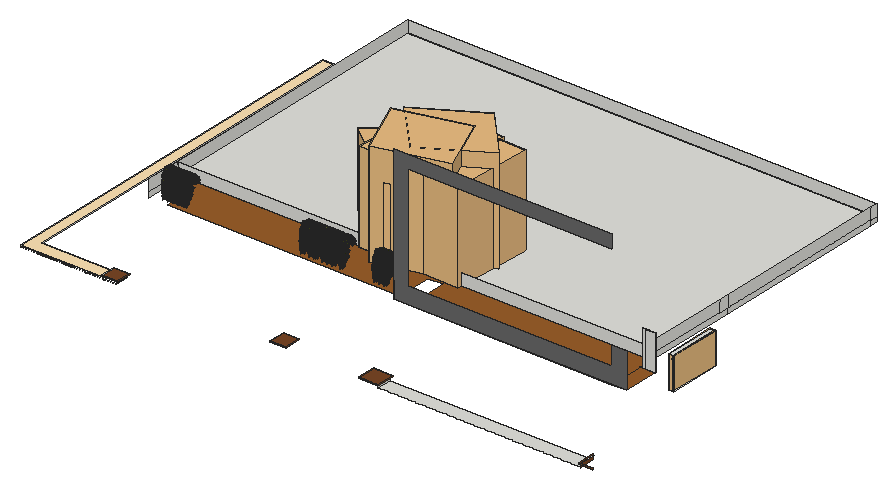
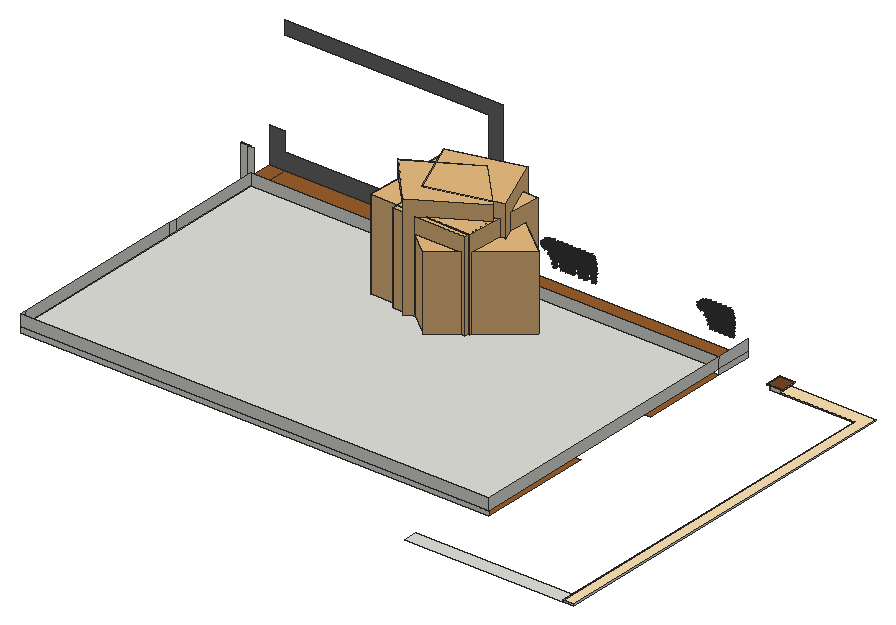
# SketchUp Ruby script. Lengths in inches.
U = 1.inch
M = Sketchup.active_model
def pt(a) = Geom::Point3d.new(a.map { |v| v * U })
def face(e, loops, mat)
  f = e.add_face(loops[0].map { |a| pt(a) })
  loops[1..].each { |l| e.add_face(l.map { |a| pt(a) }).erase! }
  f.material = f.back_material = mat if mat
  f
end
# faces: each face lists its corners as indices into pts; further lists are holes
def faces(e, pts, list, mat = nil) = list.each { |f| face(e, (f[0].is_a?(Array) ? f : [f]).map { |l| l.map { |i| pts[i] } }, mat) }
# xy, xz, yz: faces in a plane at the given z, y or x. An outline is a flat list of corners, or four numbers for a rectangle; further outlines are holes
def ring(l) = l.size == 4 ? [[l[0], l[1]], [l[2], l[1]], [l[2], l[3]], [l[0], l[3]]] : l.each_slice(2).to_a
def flat(e, list, mat, &to3) = list.each { |f| face(e, (f[0].is_a?(Array) ? f : [f]).map { |l| ring(l).map { |u, v| to3.(u, v) } }, mat) }
def xy(e, z, list, mat = nil) = flat(e, list, mat) { |x, y| [x, y, z] }
def xz(e, y, list, mat = nil) = flat(e, list, mat) { |x, z| [x, y, z] }
def yz(e, x, list, mat = nil) = flat(e, list, mat) { |y, z| [x, y, z] }
def lines(e, pts, list) = list.each { |a, b| e.add_line(pt(pts[a]), pt(pts[b])) }
# prism: a flat outline (further loops are holes) pulled along v
def prism(e, loops, v, mat = nil)
  f = face(e, loops, mat); d = Geom::Vector3d.new(v.map { |x| x * U })
  f.pushpull(f.normal.samedirection?(d) ? d.length : -d.length)
end
def box(e, o, s, mat = nil) = prism(e, [[o, [o[0] + s[0], o[1], o[2]], [o[0] + s[0], o[1] + s[1], o[2]], [o[0], o[1] + s[1], o[2]]]], [0, 0, s[2]], mat)
def at(x, y, z, deg = 0) = Geom::Transformation.translation(pt([x, y, z])) * Geom::Transformation.rotation(ORIGIN, Z_AXIS, deg.degrees)
def axes(o, x, y, z) = Geom::Transformation.new([*x, 0, *y, 0, *z, 0, *pt(o).to_a, 1])
def part(name) = M.definitions.add(name)
# library, detail: a bought-in or finely detailed component or shape, given as its bounding box
def library(name, o, s) = part(name).tap { |d| box(d.entities, o, s) }
def detail(e, o, s) = box(e.add_group.entities, o, s)
def put(e, d, t, mat = nil) = e.add_instance(d, t).tap { |i| i.material = mat if mat }
def group(e, t, mat = nil) = e.add_group.tap { |g| g.transformation = t; g.material = mat if mat }.entities
root = M.entities
M.materials.add("[0032_Moccasin]").color = [255, 228, 181]
M.materials.add("[0134_DimGray]").color = [105, 105, 105]
M.materials.add("[0136_Charcoal]").color = [35, 35, 35]
M.materials.add("[Wood Floor Dark]").color = [153, 94, 42]
M.materials.add("[Wood Veneer 01]").color = [120, 70, 37]
M.materials.add("asdfasdfasdfasdf").color = [186, 198, 91]
M.materials.add("leaf1_smaller_cleanasdfasfasdfas").color = [88, 95, 33]
M.materials.add("leaf2_smaller_cleansadfasdfasdfasd").color = [55, 66, 19]
c1 = part("leaf1a")
p = [[1.06,3.74,11.78],[8.28,8.7,-0.64],[9.51,5.4,26.1],[17.76,4.04,11.26],[17.85,2.23,20],[14.31,3.29,26.73],
  [3.78,3.8125,25.98],[-0.21,2.38,19.72]]
faces(c1.entities,p,[[0,1,2],[2,1,3],[3,4,5],[3,5,2],[6,7,0],[0,2,6]],"leaf1_smaller_cleanasdfasfasdfas")
c2 = part("leaf2a")
p = [[1.4375,3.56,10.81],[8.71,6.8,-0.73],[9.51,3.5,26.59],[16.66,3.91,9.8],[17.86,1.3,19.21],[14.9,1.58,24.92],
  [5.15,2.55,24.01],[1.29,1.87,19.875]]
faces(c2.entities,p,[[0,1,2],[2,1,3],[3,4,5],[3,5,2],[6,7,0],[0,2,6]],"leaf2_smaller_cleansadfasdfasdfasd")
c3 = part("Group\#49")
put(c3.entities,c2,axes([6.68,1.92,2.42],[-0.04671,0.11082,0.08136],[0.07715,0.09226,-0.08136],[-0.11379,0.01705,-0.08856]))
put(c3.entities,c1,axes([1.26,0.54,1.25],[0.13756,-0.04533,0.01029],[0.0079,-0.00888,-0.14471],[0.04581,0.13766,-0.00594]))
put(c3.entities,c2,axes([-0.51,4.89,1.49],[-0.00057,-0.14139,-0.03304],[0.00922,0.03294,-0.14111],[0.14491,-0.00265,0.00885]))
put(c3.entities,c1,axes([4.37,7.98,1.26],[-0.14226,-0.02905,0],[0,0,-0.1452],[0.02905,-0.14226,0]))
put(c3.entities,c1,axes([1.46,4.03,4.07],[0.06242,-0.12847,-0.02614],[-0.10319,-0.03029,-0.09755],[0.08086,0.06051,-0.10432]))
c4 = part("leaf_a")
p = [[1.43,4.41,0.74],[1.39,4.36,0.69],[1.39,4.61,0.21],[1.43,4.67,0.24],[1.35,4.41,0.74],[1.35,4.67,0.24],
  [1.35,3.9,1.02],[1.43,3.9,1.02],[1.39,3.89,0.95],[1.39,3.35,0.9],[1.43,3.34,0.96],[1.35,3.34,0.96]]
faces(c4.entities,p,[[0,1,2,3],[1,4,5,2],[4,0,3,5],[3,2,5],[6,7,0,4],[8,6,4,1],[7,8,1,0],[9,10,11],
  [9,11,6,8],[10,9,8,7],[11,10,7,6]],"asdfasdfasdfasdf")
put(c4.entities,c2,axes([0,-0.08,0.875],[0.1452,0,0],[0,0.02746,-0.14258],[0,0.14258,0.02746]))
c5 = part("leaf_b")
prism(c5.entities,[[[1.36,4.21,-0.25],[1.31,4.13,-0.29],[1.26,4.21,-0.25]]],[0,-0.66,1.14],"asdfasdfasdfasdf")
put(c5.entities,c1,axes([0,-0.1,0.68],[0.1452,-0.0002,0],[0.00006,0.04124,-0.13922],[0.00019,0.13922,0.04124]))
c6 = part("Group\#47")
p = [[2.87,4.13,4.15],[2.98,3.98,4.12],[2.98,4.66,2.59],[2.87,4.8,2.65],[3.09,4.13,4.15],[3.09,4.8,2.65],
  [2.87,4.13,6.07],[2.98,3.98,6.12],[3.09,4.13,6.07],[2.87,5.04,7.34],[2.98,4.91,7.43],[3.09,5.04,7.34]]
faces(c6.entities,p,[[0,1,2,3],[1,4,5,2],[6,7,1,0],[7,8,4,1],[9,10,7,6],[10,11,8,7]],"asdfasdfasdfasdf")
put(c6.entities,c4,axes([0.86,0.51,1.53],[0.95176,-0.27809,0.12967],[0.18405,0.85554,0.48392],[-0.24551,-0.43671,0.86545]))
put(c6.entities,c5,axes([-0.97,2.96,6.52],[0.70711,-0.61237,-0.35355],[0.70711,0.61237,0.35355],[0,-0.5,0.86603]))
put(c6.entities,c4,axes([3.23,0.39,0.41],[0.82736,0.50176,-0.25242],[-0.32519,0.79434,0.5131],[0.45796,-0.34244,0.82037]))
put(c6.entities,c4,axes([3.25,-0.58,4.78],[0.8251,0.44069,-0.35355],[-0.31829,0.8796,0.35355],[0.46679,-0.17918,0.86603]))
c7 = part("Group\#46")
p = [[1.22,4.71,2.14],[1.31,4.57,2.14],[2.16,4.71,3.79],[2.24,4.57,3.77],[1.39,4.71,2.14],[2.33,4.71,3.79],
  [1.93,3.51,6.2],[1.85,3.64,6.23],[2.02,3.64,6.23],[0.93,3.38,8.58],[0.85,3.52,8.58],[1.02,3.52,8.58],
  [0.81,3.57,10.77],[0.72,3.71,10.73],[0.89,3.71,10.73],[1.31,4.57,13.2],[1.22,4.7,13.15],[1.39,4.7,13.15]]
faces(c7.entities,p,[[0,1,2],[3,2,1],[1,4,3],[5,3,4],[6,7,3],[6,3,8],[2,3,7],[5,8,3],
  [9,10,6],[9,6,11],[7,6,10],[8,11,6],[9,11,12],[9,12,10],[13,10,12],[14,12,11],
  [12,15,13],[12,14,15],[16,13,15],[17,15,14]],"asdfasdfasdfasdf")
put(c7.entities,c5,axes([3.93,1.17,1.97],[0.75139,0.49793,0.43299],[-0.65983,0.56085,0.50006],[0.00615,-0.66145,0.74997]))
put(c7.entities,c5,axes([6.23,5.09,1.92],[-0.36585,0.92196,0.12706],[-0.79398,-0.38042,0.47421],[0.48554,0.0726,0.87119]))
put(c7.entities,c5,axes([0.03,0.92,11.26],[1,0,0],[0,0.86603,0.5],[0,-0.5,0.86603]))
put(c7.entities,c4,axes([4.37,2.0625,9.11],[0.45529,0.76896,0.44879],[-0.86129,0.25267,0.44084],[0.22559,-0.58725,0.77733]))
put(c7.entities,c4,axes([1.89,-0.25,4.42],[0.88717,0.14116,0.43931],[-0.36372,0.79981,0.47751],[-0.28396,-0.58342,0.76091]))
put(c7.entities,c4,axes([-0.4,-0.0625,7.9],[0.80178,0.42258,-0.42258],[0,0.70711,0.70711],[0.59763,-0.56694,0.56694]))
put(c7.entities,c5,axes([0.05,0.6875,0.65],[0.97178,0.10445,-0.21151],[0.0126,0.87237,0.48869],[0.23556,-0.47756,0.84643]))
put(c7.entities,c4,axes([5.56,1.19,4.08],[0.24789,0.96746,-0.05068],[-0.86286,0.24427,0.4425],[0.44048,-0.06596,0.89533]))
put(c7.entities,c5,axes([4.91,2.14,7.29],[-0.04249,0.96546,-0.25705],[-0.89911,0.07524,0.4312],[0.43565,0.24944,0.86486]))
c8 = part("Group\#48")
put(c8.entities,c2,axes([5.59,5.52,3.3],[-0.07606,0.12201,-0.02028],[0.09645,0.0436,-0.0994],[-0.07744,-0.06554,-0.10388]))
put(c8.entities,c2,axes([7.69,4.27,1.08],[-0.09839,0.10661,0.00609],[-0.00698,0.00184,-0.14502],[-0.10656,-0.09856,0.00388]))
put(c8.entities,c1,axes([3.51,6.9,2.1],[-0.1403,-0.03711,-0.00465],[-0.00046,0.01976,-0.14385],[0.03739,-0.13898,-0.01921]))
put(c8.entities,c2,axes([2.18,0.07,1.375],[0.14025,0.00096,-0.03757],[-0.03758,0.00358,-0.14021],[0,0.14515,0.00371]))
put(c8.entities,c1,axes([-0.62,2,1.16],[0.081,-0.0806,-0.00996],[0.00004,0.01411,-0.11384],[0.08122,0.08039,0.00999]))
c9 = part("Group\#221")
p = [[1.22,4.71,2.14],[1.31,4.57,2.14],[2.16,4.71,3.79],[2.24,4.57,3.77],[1.39,4.71,2.14],[2.33,4.71,3.79],
  [1.93,3.51,6.2],[1.85,3.64,6.23],[2.02,3.64,6.23],[0.93,3.38,8.58],[0.85,3.52,8.58],[1.02,3.52,8.58],
  [0.81,3.57,10.77],[0.72,3.71,10.73],[0.89,3.71,10.73],[1.31,4.57,13.2],[1.22,4.7,13.15],[1.39,4.7,13.15]]
faces(c9.entities,p,[[0,1,2],[3,2,1],[1,4,3],[5,3,4],[6,7,3],[6,3,8],[2,3,7],[5,8,3],
  [9,10,6],[9,6,11],[7,6,10],[8,11,6],[9,11,12],[9,12,10],[13,10,12],[14,12,11],
  [12,15,13],[12,14,15],[16,13,15],[17,15,14]],"asdfasdfasdfasdf")
put(c9.entities,c5,axes([3.93,1.17,1.97],[0.75139,0.49793,0.43299],[-0.65983,0.56085,0.50006],[0.00615,-0.66145,0.74997]))
put(c9.entities,c5,axes([6.23,5.09,1.92],[-0.36585,0.92196,0.12706],[-0.79398,-0.38042,0.47421],[0.48554,0.0726,0.87119]))
put(c9.entities,c5,axes([0.03,0.92,11.26],[1,0,0],[0,0.86603,0.5],[0,-0.5,0.86603]))
put(c9.entities,c4,axes([4.37,2.0625,9.11],[0.45529,0.76896,0.44879],[-0.86129,0.25267,0.44084],[0.22559,-0.58725,0.77733]))
put(c9.entities,c4,axes([1.89,-0.25,4.42],[0.88717,0.14116,0.43931],[-0.36372,0.79981,0.47751],[-0.28396,-0.58342,0.76091]))
put(c9.entities,c4,axes([-0.4,-0.0625,7.9],[0.80178,0.42258,-0.42258],[0,0.70711,0.70711],[0.59763,-0.56694,0.56694]))
put(c9.entities,c5,axes([0.05,0.6875,0.65],[0.97178,0.10445,-0.21151],[0.0126,0.87237,0.48869],[0.23556,-0.47756,0.84643]))
put(c9.entities,c4,axes([5.56,1.19,4.08],[0.24789,0.96746,-0.05068],[-0.86286,0.24427,0.4425],[0.44048,-0.06596,0.89533]))
put(c9.entities,c5,axes([4.91,2.14,7.29],[-0.04249,0.96546,-0.25705],[-0.89911,0.07524,0.4312],[0.43565,0.24944,0.86486]))
c10 = part("Trailing philodendron foliage")
put(c10.entities,c1,axes([3.65,12.52,19.68],[-0.0527,-0.13492,0.0101],[-0.03487,0.00307,-0.14092],[0.13073,-0.05357,-0.03351]))
put(c10.entities,c1,axes([5.13,11.34,20.6],[-0.03432,-0.12484,0.06572],[-0.08608,-0.03507,-0.11155],[0.11179,-0.06533,-0.06572]))
put(c10.entities,c2,axes([2.61,13.04,18.63],[0.05838,-0.12752,0.03758],[0.01564,-0.03417,-0.14025],[0.13202,0.06044,0]))
put(c10.entities,c2,axes([3.7,9.83,20.73],[-0.00129,-0.14519,0],[-0.0726,0.00064,-0.12575],[0.12574,-0.00112,-0.0726]))
put(c10.entities,c2,axes([11.375,11.11,20.23],[-0.14171,0.00126,0.03163],[-0.02867,0.05638,-0.1307],[-0.01341,-0.1338,-0.05478]))
put(c10.entities,c1,axes([2.4375,12.45,15.12],[-0.02375,-0.14324,0],[0.13106,-0.02173,-0.05859],[0.05781,-0.00958,0.13285]))
put(c10.entities,c1,axes([9.62,10.68,22.01],[0.05693,0.12487,-0.04742],[0.05061,-0.06787,-0.11796],[-0.12361,0.02972,-0.07014]))
put(c10.entities,c1,axes([11.63,16.35,20.5625],[-0.12691,-0.00762,0.07014],[-0.06947,0.03872,-0.12148],[-0.01233,-0.13973,-0.03749]))
put(c10.entities,c1,axes([12.51,17.52,17.81],[-0.1445,0.01001,0.0102],[-0.01383,-0.07182,-0.12544],[-0.0036,-0.1258,0.07242]))
put(c10.entities,c2,axes([9.09,6.34,22.72],[-0.09269,-0.05068,-0.09962],[-0.03661,0.13604,-0.03515],[0.1056,0.00268,-0.09962]))
put(c10.entities,c1,axes([4.83,12.62,22.54],[0.10783,0.09684,-0.00888],[0.09716,-0.10783,0.00397],[-0.00394,-0.00889,-0.14487]))
put(c10.entities,c1,axes([4.94,9.48,20.375],[0.01323,0.07633,0.07653],[0.10803,-0.00667,-0.01203],[-0.00375,0.07738,-0.07653]))
put(c10.entities,c2,axes([14,13.64,21.84],[-0.01852,-0.13907,0.03741],[-0.14373,0.01547,-0.01367],[0.00911,-0.03878,-0.13963]))
put(c10.entities,c2,axes([9.23,4.15,18.71],[0.14198,0.00177,-0.03038],[-0.02867,0.05638,-0.1307],[0.01021,0.13379,0.05548]))
put(c10.entities,c2,axes([5.82,4.5625,15.3],[0.13095,-0.05433,0.03137],[0.06268,0.11013,-0.07089],[0.00273,0.07747,0.12278]))
put(c10.entities,c3,axes([6.59,5.29,16.06],[1.23201,0.26412,0],[-0.26412,1.23201,0],[0,0,1.26]))
put(c10.entities,c6,axes([12.21,1.69,0.66],[-0.82914,0.03045,-0.02227],[0.02366,0.80139,0.21474],[-0.02938,-0.21389,0.80143]))
put(c10.entities,c7,axes([6.8125,1.15,7.57],[0.74375,-0.41052,0.02847],[0.41052,0.73612,-0.11],[0.02847,0.11,0.84237]))
put(c10.entities,c6,axes([-1.68,6.875,13.2],[0.5,-0.86603,0],[0.81585,0.47103,-0.33545],[0.29051,0.16773,0.94206]))
put(c10.entities,c6,axes([1.86,19.56,12.8125],[0.88164,0.4704,0.03781],[0.46333,-0.8476,-0.25863],[0.08962,-0.24554,0.96524]))
g1 = group(c10.entities,at(9.13,11.13,20.67))
put(g1,c2,axes([7.36,4.03,-0.3],[-0.05057,0.11966,-0.06487],[0.07036,-0.03625,-0.12173],[-0.11651,-0.07383,-0.04536]))
put(g1,c2,axes([8.4,1.56,-2.35],[-0.06703,0.12496,-0.03122],[-0.04831,-0.05702,-0.12449],[-0.1194,-0.04708,0.0679]))
put(g1,c1,axes([5.37,5.58,-2.1],[-0.14013,0.0124,0.03596],[-0.03803,-0.04347,-0.13322],[-0.00061,-0.13798,0.0452]))
put(g1,c2,axes([2.45,-0.07,0.8],[0.12002,-0.06072,-0.05468],[-0.07506,-0.04353,-0.11642],[0.03229,0.1245,-0.06737]))
put(g1,c1,axes([0.19,2.38,0.125],[0.05529,-0.09889,0.01797],[-0.03005,-0.03583,-0.10474],[0.09591,0.04578,-0.04318]))
put(c10.entities,c8,axes([17.33,10.54,16.15],[-0.62797,0.46654,0.62289],[-0.59637,-0.80271,0],[0.5,-0.37147,0.78231]))
put(c10.entities,c3,axes([3.44,11.88,17.73],[0.78616,-0.36326,0.5],[0.52263,0.82256,-0.22414],[-0.32986,0.43753,0.83652]))
put(c10.entities,c8,axes([5.5,5.07,16.54],[0.96593,-0.11102,0.2338],[0,0.90334,0.42894],[-0.25882,-0.41432,0.87255]))
put(c10.entities,c6,axes([18.84,3.62,12.91],[-0.80696,-0.59061,0],[-0.57048,0.77946,-0.25882],[-0.15286,0.20886,0.96593]))
put(c10.entities,c7,axes([3.89,0.96,5.21],[0.83948,0.00528,-0.02906],[-0.009,0.83292,-0.10846],[0.02813,0.1087,0.83246]))
put(c10.entities,c7,axes([6.1,0.84,-5.33],[0.875,-0.48296,0.03349],[0.48296,0.86603,-0.12941],[0.03349,0.12941,0.99103]))
put(c10.entities,c7,axes([3.87,-0.55,-8.84],[0.99938,0.00629,-0.0346],[-0.01071,0.99157,-0.12912],[0.03349,0.12941,0.99103]))
put(c10.entities,c6,axes([0.46,6.875,13.01],[0.5,-0.86603,0],[0.81585,0.47103,-0.33545],[0.29051,0.16773,0.94206]))
put(c10.entities,c7,axes([10.39,0.84,1.73],[0.875,-0.48296,0.03349],[0.48296,0.86603,-0.12941],[0.03349,0.12941,0.99103]))
put(c10.entities,c7,axes([-0.75,1.13,2.67],[0.7525,-0.41535,0.0288],[0.41535,0.74478,-0.11129],[0.0288,0.11129,0.85228]))
put(c10.entities,c7,axes([0.04,-0.97,-8.67],[0.735,-0.40569,0.02813],[0.40569,0.72746,-0.1087],[0.02813,0.1087,0.83246]))
put(c10.entities,c7,axes([0.09,-0.6,-7.42],[0.47403,-0.32078,-0.33698],[0.20171,0.57521,-0.26383],[0.41925,0.08595,0.50794]))
put(c10.entities,c7,axes([10.35,0.97,-6.0625],[0.76125,-0.42018,0.02914],[0.42018,0.75344,-0.11259],[0.02914,0.11259,0.86219]))
put(c10.entities,c7,axes([10.78,-1.55,-11.77],[0.72777,-0.42018,0.22517],[0.435,0.75344,0],[-0.19501,0.11259,0.84036]))
put(c10.entities,c7,axes([5.78,-1.55,-20.23],[0.76125,-0.42018,0.02914],[0.42018,0.75344,-0.11259],[0.02914,0.11259,0.86219]))
put(c10.entities,c7,axes([8.72,-1.43,-13.97],[0.65467,-0.36135,0.02506],[0.36135,0.64796,-0.09682],[0.02506,0.09682,0.74149]))
put(c10.entities,c9,axes([1.53,-0.97,-19.86],[0.735,-0.40569,0.02813],[0.40569,0.72746,-0.1087],[0.02813,0.1087,0.83246]))
put(c10.entities,c9,axes([6.23,-2.02,-7.18],[0.55125,-0.30427,0.0211],[0.39555,0.70927,-0.10599],[0.0211,0.08153,0.62435]))
put(c10.entities,c9,axes([6.43,-1.89,6.18],[0.735,-0.40569,0.02813],[0.5274,0.9457,-0.14132],[0.02813,0.1087,0.83246]))
put(c10.entities,c9,axes([10.24,1.09,9.64],[0.62475,-0.34484,0.02391],[0.44829,0.80384,-0.12012],[0.02391,0.0924,0.70759]))
put(c10.entities,c6,axes([1.56,7.74,12.8125],[-0.22619,0.97335,0.03781],[0.93864,0.22817,-0.25863],[0.26037,0.02301,0.96524]))
put(c10.entities,c6,axes([0.65,14.36,12.8125],[0.30411,0.95189,0.03781],[0.92309,-0.28464,-0.25863],[0.23543,-0.11355,0.96524]))
put(c10.entities,c6,axes([7.75,10.38,12.8125],[-0.84074,0.54011,0.03781],[0.51385,0.81797,-0.25863],[0.17062,0.19802,0.96524]))
put(c10.entities,c6,axes([12.92,19.16,12.8125],[0.9234,-0.38197,0.03781],[-0.36017,-0.89632,-0.25863],[-0.13268,-0.22521,0.96524]))
put(c10.entities,c6,axes([6.55,17.22,12.8125],[0.7985,0.60081,0.03781],[0.58857,-0.76596,-0.25863],[0.12643,-0.22877,0.96524]))
put(c10.entities,c6,axes([16.24,8.94,12.8125],[-0.64953,-0.75939,0.03781],[-0.7404,0.62041,-0.25863],[-0.17295,0.19599,0.96524]))
put(c10.entities,c6,axes([15.6875,15.74,12.8125],[0.12972,-0.99083,0.03781],[-0.95648,-0.13509,-0.25863],[-0.26137,0.00261,0.96524]))
put(c10.entities,c6,axes([19.85,8,15.61],[-0.64953,-0.75939,0.03781],[-0.7404,0.62041,-0.25863],[-0.17295,0.19599,0.96524]))
put(c10.entities,c6,axes([18.86,17.5,12.8125],[0.62831,-0.77705,0.03781],[-0.74495,-0.61494,-0.25863],[-0.22422,-0.13434,0.96524]))
put(c10.entities,c6,axes([-0.43,13.28,13.2],[-0.41945,-0.90778,0],[0.85518,-0.39515,-0.33545],[0.30452,-0.14071,0.94206]))
put(c10.entities,c9,axes([4.5625,-2.01,7.45],[0.56595,-0.31238,0.02166],[0.40609,0.72819,-0.10881],[0.02166,0.0837,0.641]))
put(c10.entities,c9,axes([4.48,-2.02,-24.24],[0.55125,-0.30427,0.0211],[0.39555,0.70927,-0.10599],[0.0211,0.08153,0.62435]))
put(c10.entities,c9,axes([4.9,-4.23,-11.04],[0.55125,-0.30427,0.0211],[0.39555,0.70927,-0.10599],[0.0211,0.08153,0.62435]))
put(c10.entities,c8,axes([17.33,10.54,17.41],[-0.62797,0.46654,0.62289],[-0.59637,-0.80271,0],[0.5,-0.37147,0.78231]))
put(c10.entities,c6,axes([-0.03,6.82,20.63],[0.44714,-0.87214,-0.19857],[0.53417,0.43844,-0.7228],[0.71744,0.21712,0.66191]))
put(c10.entities,c6,axes([20.82,12.8,12.8125],[0.12972,-0.99083,0.03781],[-0.95648,-0.13509,-0.25863],[-0.26137,0.00261,0.96524]))
c11 = library("Group\#40",[-33.32,-34.9375,32.67],[162.87,159.66,128.34])
c12 = library("Group\#43",[-10.45,-6.67,0],[121.7,116.61,164.95])
c13 = library("Group\#44",[-10.45,-6.67,0],[121.7,116.61,164.95])
c14 = library("Group\#41",[-10.45,-6.67,0],[121.7,116.61,164.95])
c15 = library("Group\#45",[-33.32,-34.9375,32.67],[162.87,159.66,128.34])
c16 = library("Group\#39",[-33.32,-34.9375,81.35],[162.87,159.66,79.66])
c17 = library("Group\#42",[-33.32,-34.9375,77.91],[162.87,159.66,83.1])
c18 = part("Palem Elek")
put(c18.entities,c11,axes([92.2,20.3,-29.73],[0.70711,0.70711,0],[-0.70711,0.70711,0],[0,0,0.91208]))
put(c18.entities,c12,axes([60.27,20.78,0],[1,0,0],[0,1,0],[0,0,0.85762]))
put(c18.entities,c13,at(25.45,60.83,0,-53.5))
put(c18.entities,c14,at(84.4375,135.48,0,-161.4))
put(c18.entities,c15,axes([38.54,105.7,-36.19],[-0.04013,-0.99919,0],[0.99919,-0.04013,0],[0,0,1.11001]))
put(c18.entities,c16,axes([57.15,96.51,-54.45],[-0.02003,-0.49872,0.02965],[0.4996,-0.02007,0],[0.00123,0.03065,0.51628]))
put(c18.entities,c17,axes([74.94,50.39,-54.06],[0.40095,0.29715,0.03075],[-0.29654,0.38966,0.10114],[0.04012,-0.11026,0.54246]))
c19 = part("palem elek\#1")
put(c19.entities,c18,at(-81.14,-74.56,-0.83))
c20 = part("Coqueiro")
put(c20.entities,c19,axes([83.17,89.39,9.5625],[0,1.1016,0],[-1.377,0,0],[0,0,1.39284]))
c21 = library("Klein+raam",[128.36,12.7,0],[19.68,5.51,55.12])
xy(root,66.6875,[[645.84,332.43,649.1,332.43,649.1,333.31,649.97,333.31,649.97,332.43,653.22,332.43,653.22,333.31,654.09,333.31,654.09,332.43,657.35,332.43,657.35,333.31,658.22,333.31,658.22,332.43,661.47,332.43,661.47,333.31,662.34,333.31,662.34,332.43,665.6,332.43,665.6,333.31,666.47,333.31,666.47,332.43,669.72,332.43,669.72,333.31,669.83,333.31,669.83,349.54,427.22,349.54,427.22,332.62,430.47,332.62,430.47,333.31,431.34,333.31,431.34,332.62,434.6,332.62,434.6,333.31,435.47,333.31,435.47,332.62,438.72,332.62,438.72,333.31,439.59,333.31,439.59,332.62,442.85,332.62,442.85,333.31,443.72,333.31,443.72,332.62,446.97,332.62,446.97,333.31,447.84,333.31,447.84,332.62,451.1,332.62,451.1,333.31,451.97,333.31,451.97,332.62,455.22,332.62,455.22,333.31,456.09,333.31,456.09,332.56,459.35,332.56,459.35,333.31,460.22,333.31,460.22,332.62,463.47,332.62,463.47,333.31,464.34,333.31,464.34,332.56,467.6,332.56,467.6,333.31,468.47,333.31,468.47,332.49,471.72,332.49,471.72,333.31,472.59,333.31,472.59,332.56,475.85,332.56,475.85,333.31,476.72,333.31,476.72,332.62,479.97,332.62,479.97,333.31,480.84,333.31,480.84,332.62,484.1,332.62,484.1,333.31,484.97,333.31,484.97,332.62,488.22,332.62,488.22,333.31,489.09,333.31,489.09,332.62,492.35,332.62,492.35,333.31,493.22,333.31,493.22,332.62,496.47,332.62,496.47,333.31,497.34,333.31,497.34,332.62,500.6,332.62,500.6,333.31,501.47,333.31,501.47,332.62,504.72,332.62,504.72,333.31,505.59,333.31,505.59,332.62,508.85,332.62,508.85,333.31,509.72,333.31,509.72,332.62,512.97,332.62,512.97,333.31,513.84,333.31,513.84,332.62,517.1,332.62,517.1,333.31,517.97,333.31,517.97,332.62,521.22,332.62,521.22,333.31,522.09,333.31,522.09,332.62,525.35,332.62,525.35,333.31,526.22,333.31,526.22,332.62,529.47,332.62,529.47,333.31,530.34,333.31,530.34,332.62,533.6,332.62,533.6,333.31,534.47,333.31,534.47,332.62,537.72,332.62,537.72,333.31,538.59,333.31,538.59,332.62,541.85,332.62,541.85,333.31,542.72,333.31,542.72,332.62,545.97,332.62,545.97,333.31,546.84,333.31,546.84,332.62,550.1,332.62,550.1,333.31,550.97,333.31,550.97,332.62,554.22,332.62,554.22,333.31,555.09,333.31,555.09,332.62,558.35,332.62,558.35,333.31,559.22,333.31,559.22,332.62,562.47,332.62,562.47,333.31,563.34,333.31,563.34,332.62,566.6,332.62,566.6,333.31,567.47,333.31,567.47,332.62,570.72,332.62,570.72,333.31,571.59,333.31,571.59,332.62,574.85,332.62,574.85,333.31,575.72,333.31,575.72,332.62,578.97,332.62,578.97,333.31,579.84,333.31,579.84,332.62,583.1,332.62,583.1,333.31,583.97,333.31,583.97,332.62,587.22,332.62,587.22,333.31,588.09,333.31,588.09,332.62,591.35,332.62,591.35,333.31,592.22,333.31,592.22,332.62,595.47,332.62,595.47,333.31,596.34,333.31,596.34,332.62,599.6,332.62,599.6,333.31,600.47,333.31,600.47,332.62,603.72,332.62,603.72,333.31,604.59,333.31,604.59,332.62,607.85,332.62,607.85,333.31,608.72,333.31,608.72,332.62,611.97,332.62,611.97,333.31,612.84,333.31,612.84,332.62,616.1,332.62,616.1,333.31,616.97,333.31,616.97,332.62,620.22,332.62,620.22,333.31,621.09,333.31,621.09,332.62,624.35,332.62,624.35,333.31,625.22,333.31,625.22,332.62,628.47,332.62,628.47,333.31,629.34,333.31,629.34,332.62,632.6,332.62,632.6,333.31,633.47,333.31,633.47,332.62,636.72,332.62,636.72,333.31,637.59,333.31,637.59,332.62,640.85,332.62,640.85,333.31,641.72,333.31,641.72,332.62,644.97,332.62,644.97,333.31,645.84,333.31],[0,333.31,20.04,334.06],[20.86,333.31,40.09,334.06],[40.9,333.31,60.13,334.06],[60.95,333.31,80.18,334.06],
  [80.99,333.31,100.22,334.06],[101.04,333.31,114.2,334.06],[12.79,768.3,201.625,784.05]])
xy(root,68.25,[[0,334.06,101.1875,334.06,101.1875,349.54,12.79,349.54,12.79,784.05,0,784.05]],"[0032_Moccasin]")
xy(root,70.8125,[[406.86,329.68,408.98,351.48],[408.98,329.68,408.98,331.81,427.22,331.81,427.22,333.31,429.28,333.31,429.28,329.68],[668.33,330.31,669.83,333.31],[669.83,330.31,683.8,331.81],[99.0625,331.18,117.08,334.06],
  [298.96,331.18,298.96,332.68,315.7,332.68,315.7,333.31,317.82,333.31,317.82,331.18],[408.98,331.81,427.22,349.54],[298.96,332.68,315.7,349.54],[315.7,333.31,317.82,351.67],[427.22,333.31,429.28,351.48],
  [668.33,333.31,669.83,351.04],[99.0625,334.06,101.1875,349.54],[101.1875,334.06,114.2,349.54],[114.2,334.06,117.08,349.54],[298.96,349.54,301.08,351.67],
  [301.08,349.54,315.7,351.67],[408.98,349.54,427.22,351.48]])
xy(root,72,[[406.86,329.68,429.28,351.48],[99.0625,331.18,117.08,349.54],[298.96,331.18,317.82,351.67]],"[Wood Veneer 01]")
xy(root,84.24,[[660.05,474.23,666.61,536.02]])
xy(root,117.59,[[446,551.1875,524.68,562.07]])
xy(root,118.5,[[303.76,551.1875,363.88,562.07]])
xy(root,122.43,[[660.05,474.23,666.61,536.02]])
xy(root,126.6875,[[666.61,431.86,666.61,432.17,669.16,432.17,669.16,433.11,671.28,433.11,671.28,432.17,677.84,432.17,677.84,433.11,678.11,433.11,678.11,431.86],[666.61,432.17,669.16,433.11],[671.28,432.17,677.84,433.11],[201.625,551.1875,201.625,784.05,660.05,784.05,660.05,775.6875,209.98,775.6875,209.98,562.07,660.05,562.07,660.05,551.1875],[209.98,562.07,660.05,775.6875]])
xy(root,126.6875,[[[400.76,389.67,400.76,397.92,418.84,397.92,418.84,440.22,400.76,440.22,400.76,397.92,124.125,397.92,124.125,440.22,101.6875,440.22,101.6875,542.92,121.5,542.92,121.5,569.92,126.375,569.92,126.375,646.79,101.6875,646.79,101.6875,784.05,201.625,784.05,201.625,551.1875,660.05,551.1875,660.05,389.67],[192.11,506.17,199.48,517.35],[171.55,506.17,177.8,517.35]],[660.05,389.67,678.11,431.86]],"[Wood Floor Dark]")
xy(root,132.6875,[[101.6875,440.22,660.05,784.05]])
xz(root,329.68,[[406.86,70.8125,429.28,72]],"[Wood Veneer 01]")
xz(root,330.31,[[668.33,70.8125,685.3,72]],"[Wood Veneer 01]")
xz(root,331.18,[[99.0625,70.8125,117.08,72],[298.96,70.8125,317.82,72]],"[Wood Veneer 01]")
xz(root,349.54,[[12.79,66.6875,12.79,68.25,101.1875,68.25,101.1875,70.8125,114.2,70.8125,114.2,66.6875],[99.0625,70.8125,117.08,72]])
xz(root,351.48,[[406.86,70.8125,429.28,72]])
xz(root,351.67,[[298.96,70.8125,317.82,72]])
xz(root,389.67,[[400.76,126.6875,678.11,126.6875,678.11,169.25,660.05,169.25,660.05,146.375,416.52,146.375,416.52,271.24,660.05,271.24,660.05,287.5625,400.76,287.5625]],"[0134_DimGray]")
xz(root,431.86,[[666.61,126.6875,678.11,169.25]])
xz(root,433.11,[[662.59,126.6875,669.16,169.25],[671.28,126.6875,677.84,169.25]])
xz(root,440.22,[[101.6875,132.6875,660.05,146.375]])
xz(root,474.23,[[660.05,84.24,666.61,122.43]])
xz(root,536.02,[[660.05,84.24,666.61,122.43]])
xz(root,784.05,[[0,66.6875,12.79,68.25],[101.6875,126.6875,660.05,132.6875],[101.6875,132.6875,660.05,146.375]])
yz(root,0,[[334.06,66.6875,784.05,68.25]])
yz(root,12.79,[[349.54,66.6875,768.3,68.25],[768.3,66.6875,784.05,68.25]])
yz(root,99.0625,[[331.18,70.8125,349.54,72]])
yz(root,101.1875,[[334.06,68.25,349.54,70.8125]])
yz(root,101.6875,[[397.92,126.6875,440.22,132.6875],[397.92,132.6875,440.22,146.375],[440.22,132.6875,784.05,146.375]])
yz(root,114.2,[[334.06,66.6875,349.54,70.8125]],"[0136_Charcoal]")
yz(root,117.08,[[331.18,70.8125,349.54,72]],"[Wood Veneer 01]")
yz(root,298.96,[[331.18,70.8125,351.67,72]],"[Wood Veneer 01]")
yz(root,317.82,[[331.18,70.8125,351.67,72]],"[Wood Veneer 01]")
yz(root,400.76,[[389.67,126.6875,397.92,132.6875],[389.67,132.6875,397.92,146.375]])
yz(root,406.86,[[329.68,70.8125,351.48,72]],"[Wood Veneer 01]")
yz(root,427.22,[[331.81,66.6875,349.54,70.8125]])
yz(root,429.28,[[329.68,70.8125,351.48,72]],"[Wood Veneer 01]")
yz(root,660.05,[[440.22,126.6875,562.07,132.6875],[562.07,126.6875,775.6875,132.6875],[775.6875,126.6875,784.05,132.6875],[440.22,132.6875,551.1875,146.375],[551.1875,132.6875,562.07,146.375],
  [562.07,132.6875,775.6875,146.375],[775.6875,132.6875,784.05,146.375]])
yz(root,668.33,[[330.31,70.8125,351.04,72]],"[Wood Veneer 01]")
yz(root,669.83,[[331.81,66.6875,349.54,70.8125]],"[Wood Veneer 01]")
p = [[660.05,440.22,132.6875],[660.05,431.86,132.6875]]
lines(root,p,[[0,1]])
put(root,c10,axes([121.31,391.41,153.43],[0.69913,-0.08089,0],[0.08089,0.69913,0],[0,0,0.70379]))
put(root,c10,axes([127.31,391.41,153.43],[0.69913,-0.08089,0],[0.08089,0.69913,0],[0,0,0.70379]))
put(root,c10,axes([133.31,391.41,153.43],[0.69913,-0.08089,0],[0.08089,0.69913,0],[0,0,0.70379]))
put(root,c10,axes([139.31,391.41,153.43],[0.69913,-0.08089,0],[0.08089,0.69913,0],[0,0,0.70379]))
put(root,c10,axes([145.31,391.41,153.43],[0.69913,-0.08089,0],[0.08089,0.69913,0],[0,0,0.70379]))
put(root,c10,axes([285.79,391.41,153.43],[0.69913,-0.08089,0],[0.08089,0.69913,0],[0,0,0.70379]))
put(root,c10,axes([295.29,391.41,153.43],[0.69913,-0.08089,0],[0.08089,0.69913,0],[0,0,0.70379]))
put(root,c10,axes([301.29,391.41,153.43],[0.69913,-0.08089,0],[0.08089,0.69913,0],[0,0,0.70379]))
put(root,c10,axes([310.6,391.41,153.43],[0.69913,-0.08089,0],[0.08089,0.69913,0],[0,0,0.70379]))
put(root,c10,axes([316.6,391.41,153.43],[0.69913,-0.08089,0],[0.08089,0.69913,0],[0,0,0.70379]))
put(root,c10,axes([322.6,391.41,153.43],[0.69913,-0.08089,0],[0.08089,0.69913,0],[0,0,0.70379]))
put(root,c10,axes([331.67,391.41,153.43],[0.69913,-0.08089,0],[0.08089,0.69913,0],[0,0,0.70379]))
put(root,c20,axes([323.05,436.33,127.77],[0.54,0,0],[0,0.54,0],[0,0,0.54]))
put(root,c10,axes([372.37,391.41,153.43],[0.69913,-0.08089,0],[0.08089,0.69913,0],[0,0,0.70379]))
put(root,c10,axes([378.37,391.41,153.43],[0.69913,-0.08089,0],[0.08089,0.69913,0],[0,0,0.70379]))
put(root,c10,axes([384.17,391.41,153.43],[0.69913,-0.08089,0],[0.08089,0.69913,0],[0,0,0.70379]))
put(root,c21,axes([647.35,474.23,-164.77],[0,0,1.93992],[1,0,0],[0,1.12102,0]))
